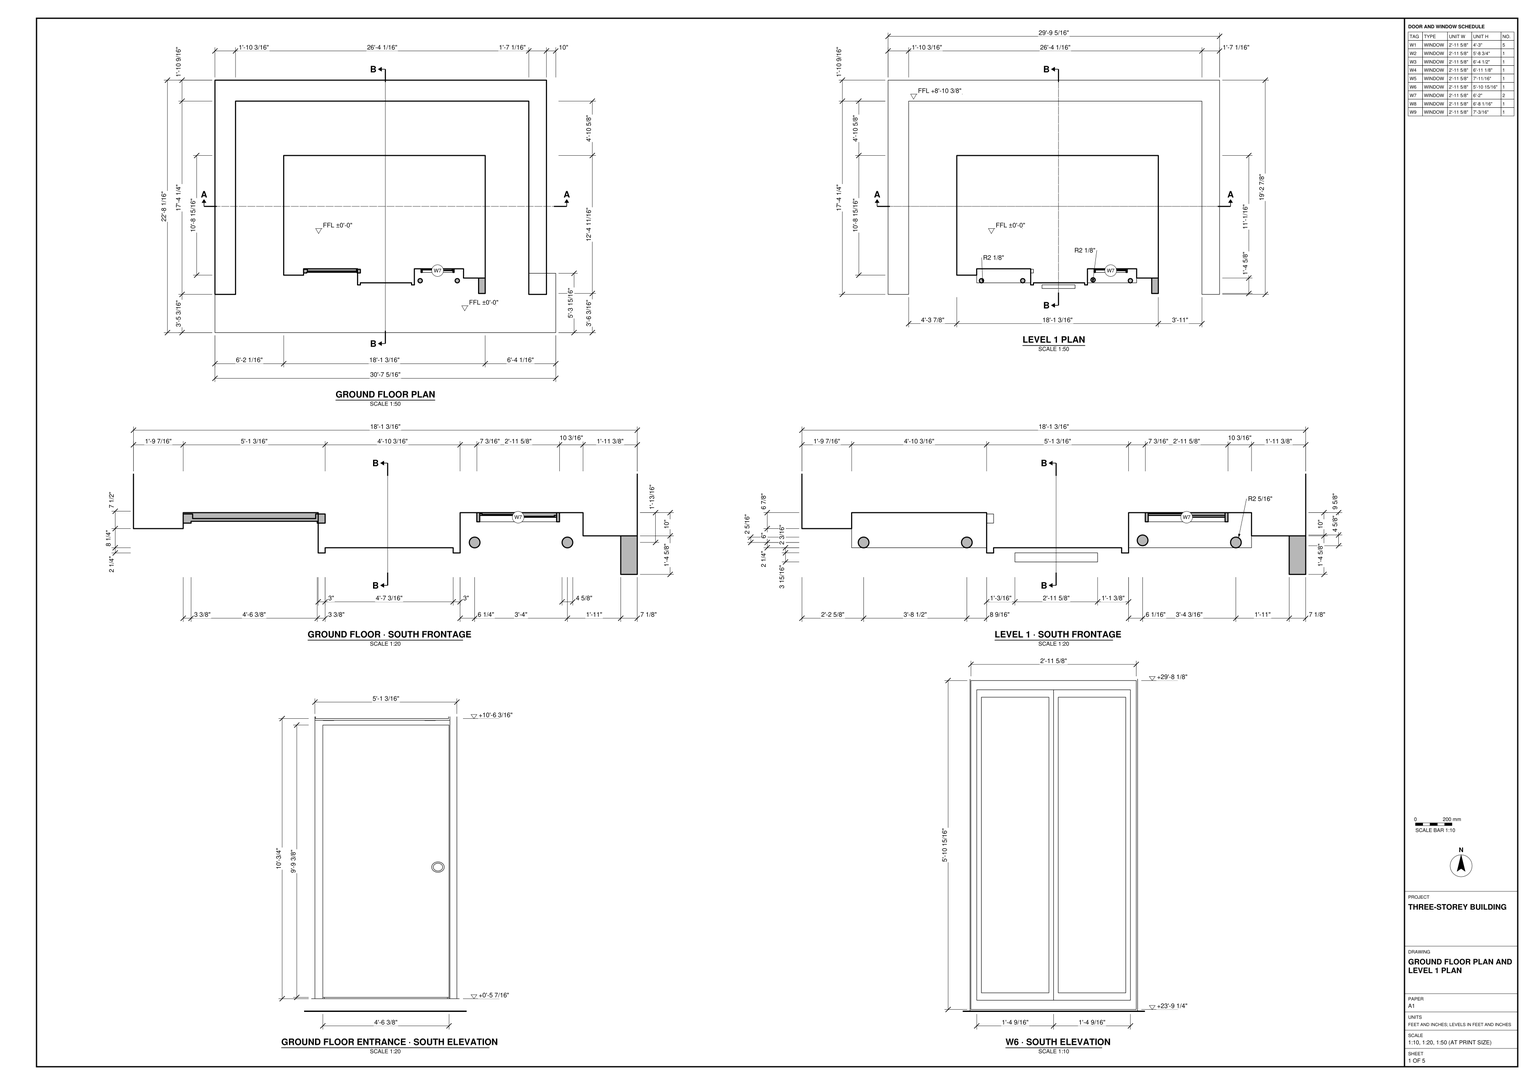
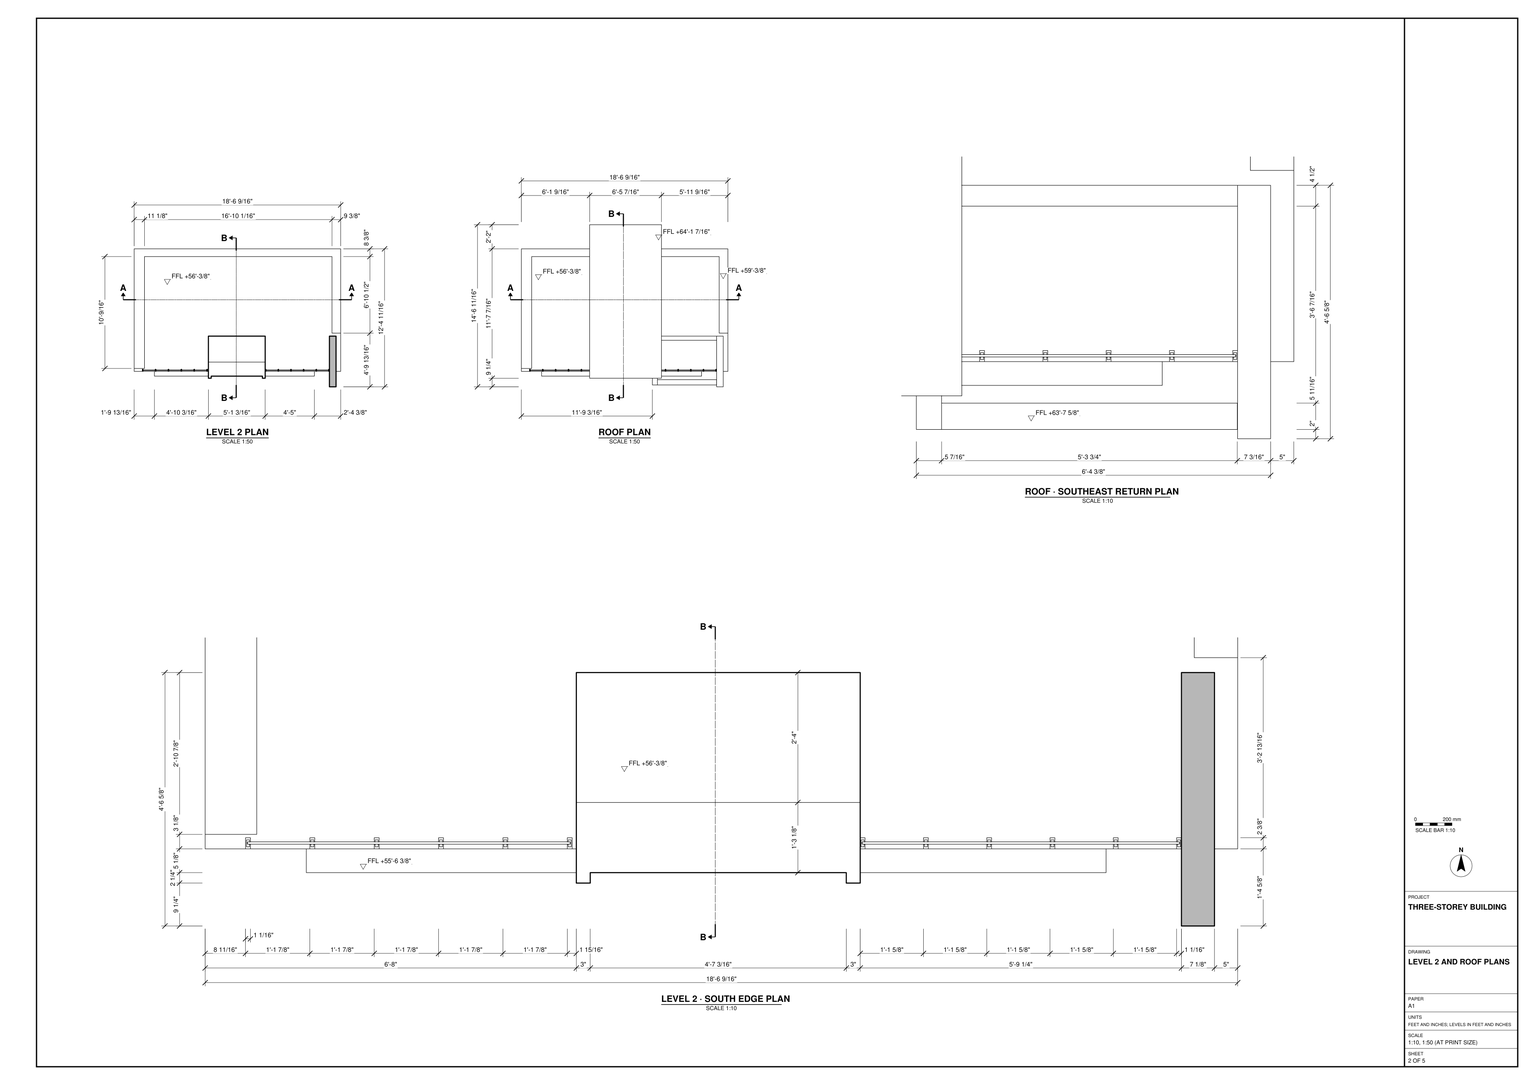
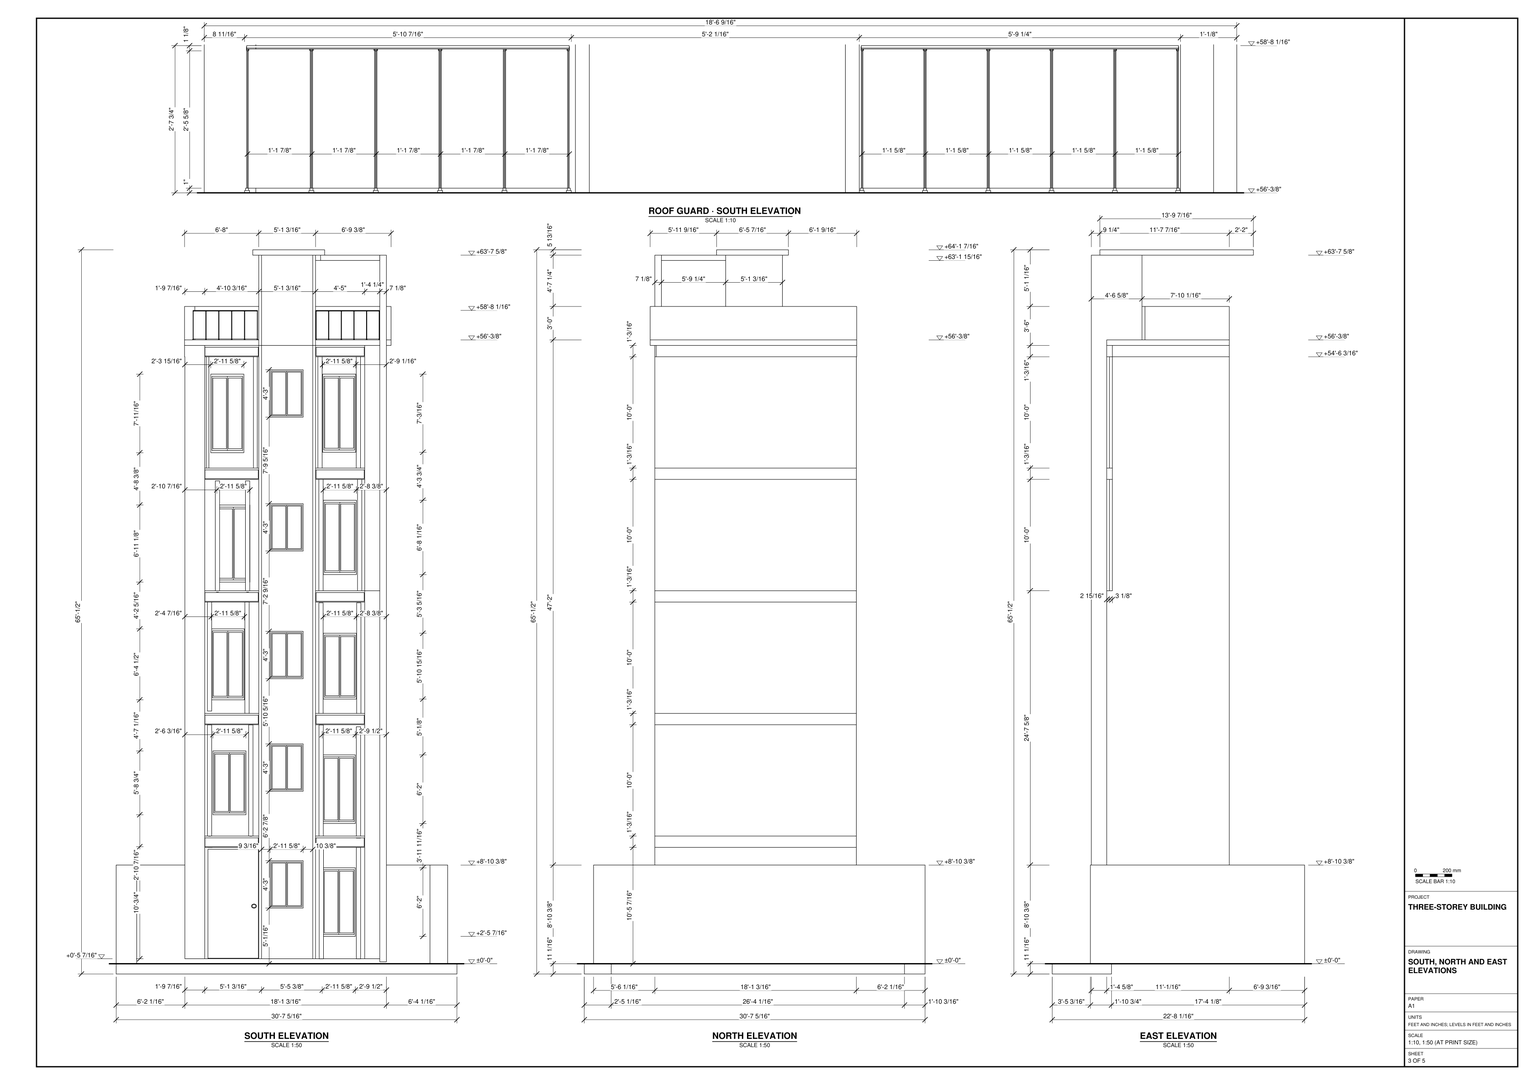
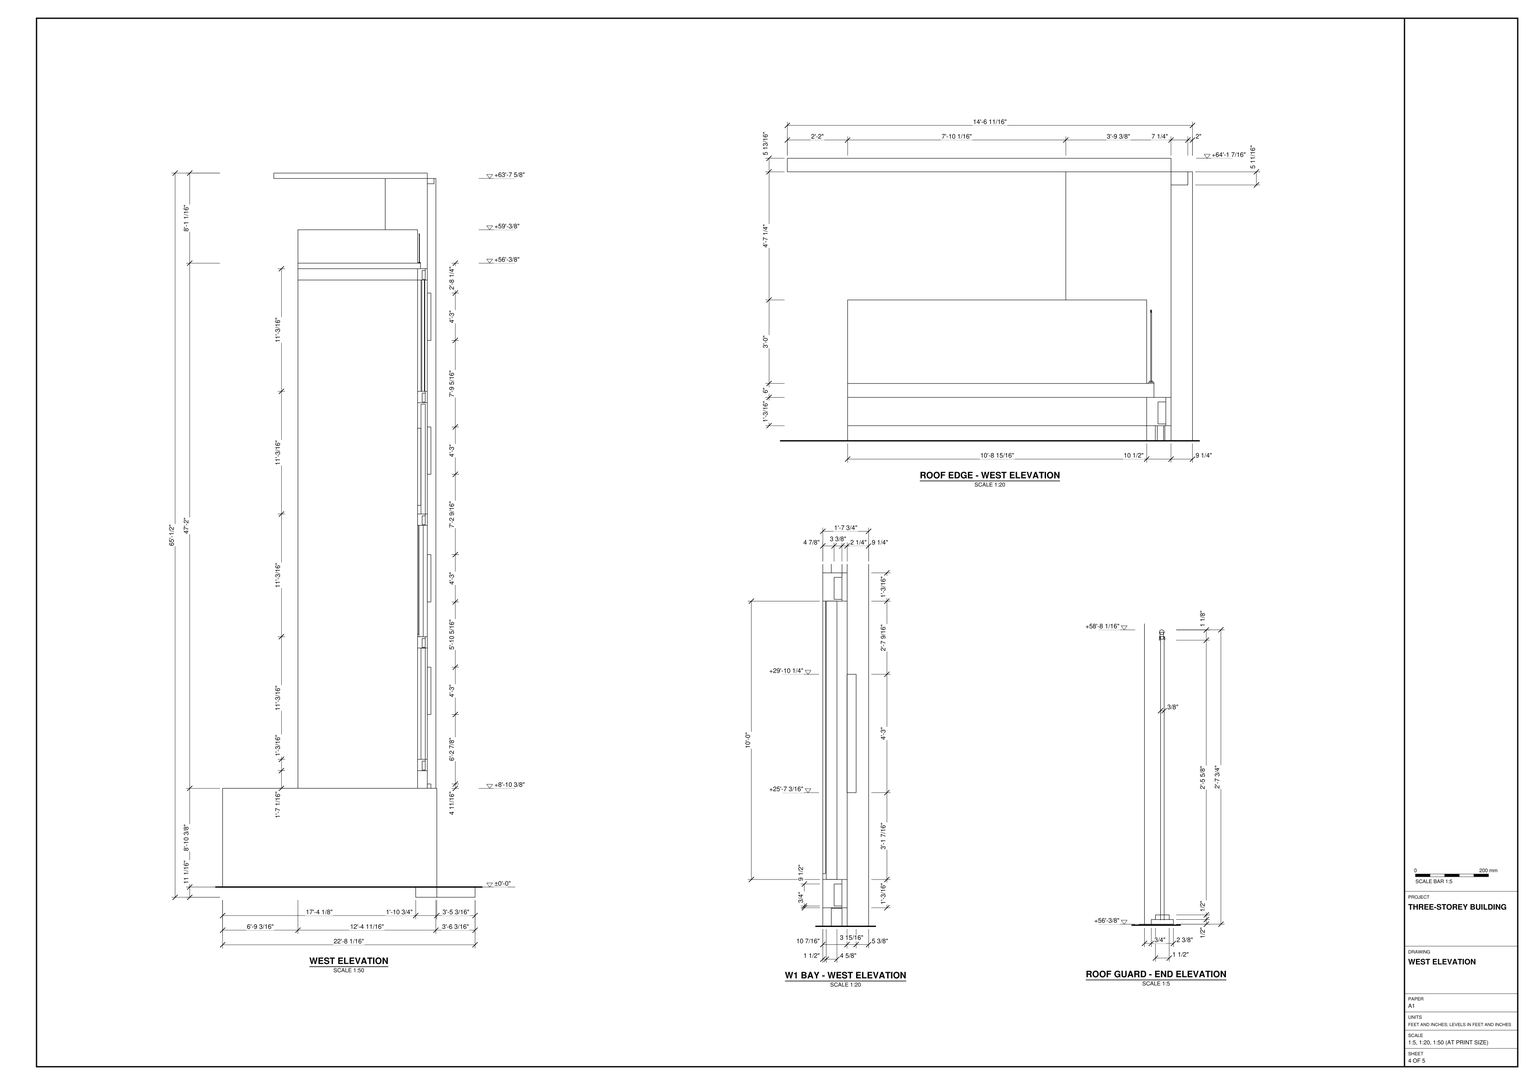
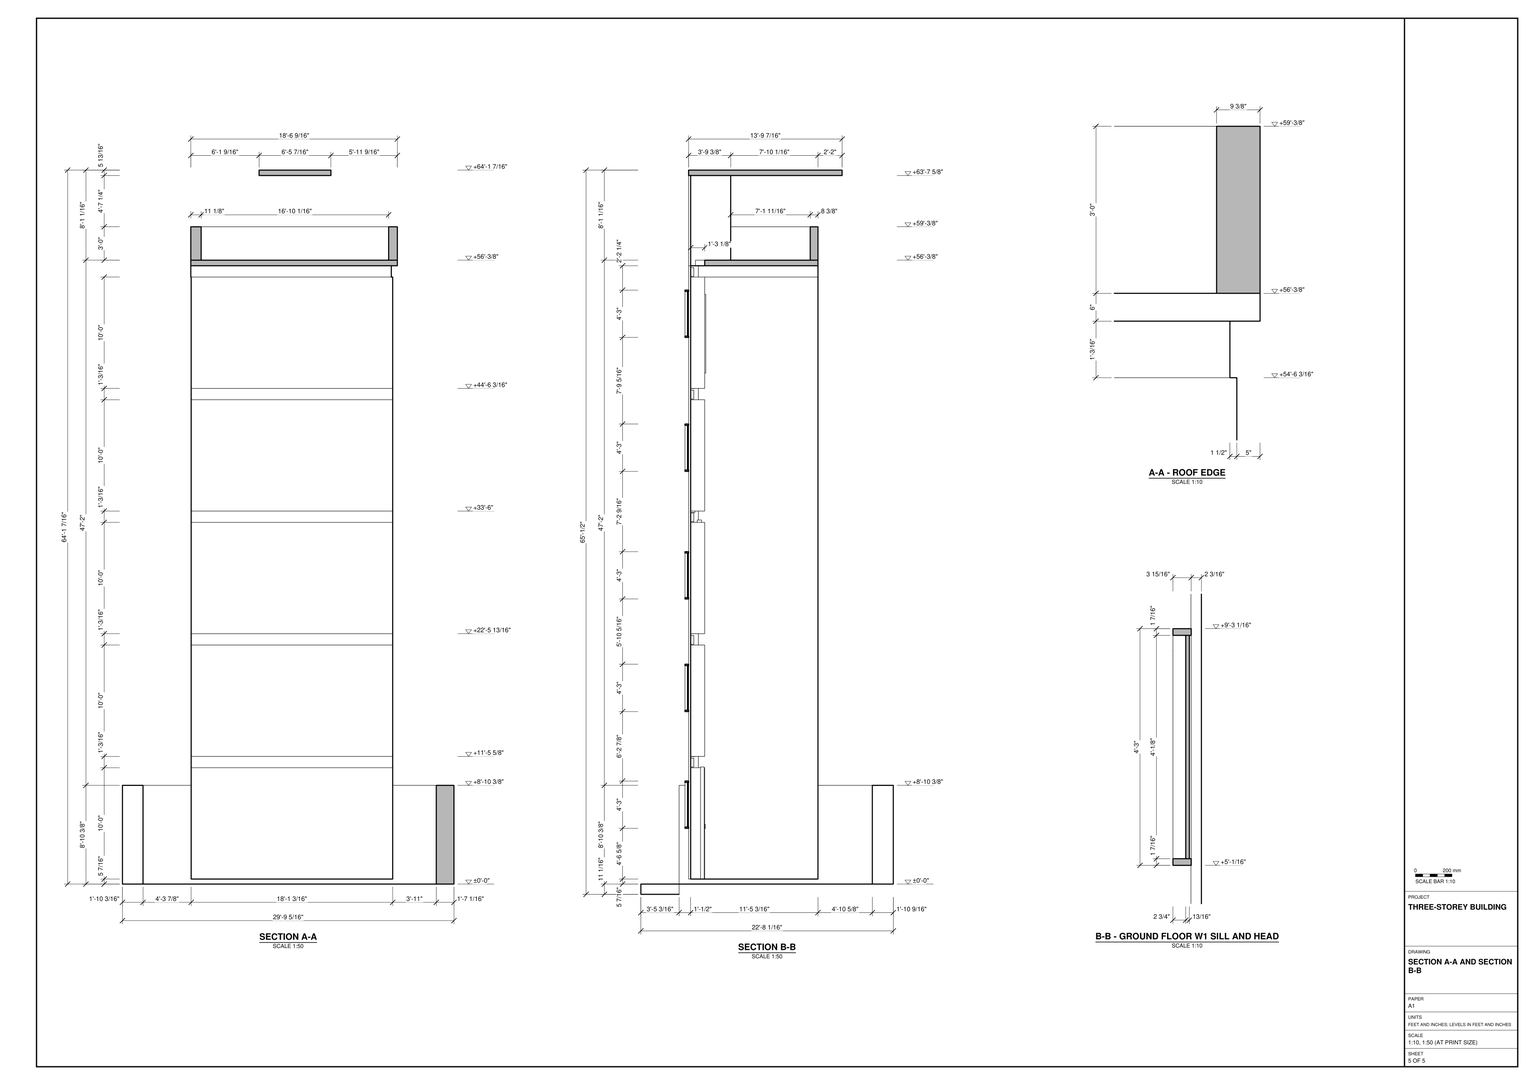
Build the building shown in task_files/diagram_01.pdf in SketchUp. Work in feet and inches. Set the overall width to 30'-7 5/16", the depth to 22'-8 1/16" and the height to 65'-1/2". Use ±0'-0" for the ground floor, +8'-10 3/8" for Level 1 and +56'-3/8" for Level 2.

Start with the ground slab and the U-shaped perimeter wall, leaving the south side open. Position the narrower building block within this surround using the offsets in plan. Follow the drawn wall thicknesses and slab edges. Use the enlarged frontage plans to set the depth of the projecting central bay and the recesses on either side. Place the entrance in the left bay as seen in the south elevation. Match the window rows, sill and head positions, frames and glazing divisions to that elevation. Use the roof plan and southeast return detail to shape the roof overhangs, and fit the glass guards on either side of the raised central bay.

Keep walls, slabs and roof elements in separate groups or components. Keep each furniture or joinery piece shown separate, and use components for repeated parts. Decor and loose items may be any suitable library components. Save one SketchUp model as output_files/three_storey_building_with_a_stepped_south_frontage.skp.

# SketchUp Ruby script. Lengths in inches.
U = 1.inch
M = Sketchup.active_model
def pt(a) = Geom::Point3d.new(a.map { |v| v * U })
def face(e, loops, mat)
  f = e.add_face(loops[0].map { |a| pt(a) })
  loops[1..].each { |l| e.add_face(l.map { |a| pt(a) }).erase! }
  f.material = f.back_material = mat if mat
  f
end
# faces: each face lists its corners as indices into pts; further lists are holes
def faces(e, pts, list, mat = nil) = list.each { |f| face(e, (f[0].is_a?(Array) ? f : [f]).map { |l| l.map { |i| pts[i] } }, mat) }
# xy, xz, yz: faces in a plane at the given z, y or x. An outline is a flat list of corners, or four numbers for a rectangle; further outlines are holes
def ring(l) = l.size == 4 ? [[l[0], l[1]], [l[2], l[1]], [l[2], l[3]], [l[0], l[3]]] : l.each_slice(2).to_a
def flat(e, list, mat, &to3) = list.each { |f| face(e, (f[0].is_a?(Array) ? f : [f]).map { |l| ring(l).map { |u, v| to3.(u, v) } }, mat) }
def xy(e, z, list, mat = nil) = flat(e, list, mat) { |x, y| [x, y, z] }
def xz(e, y, list, mat = nil) = flat(e, list, mat) { |x, z| [x, y, z] }
def yz(e, x, list, mat = nil) = flat(e, list, mat) { |y, z| [x, y, z] }
def lines(e, pts, list) = list.each { |a, b| e.add_line(pt(pts[a]), pt(pts[b])) }
# prism: a flat outline (further loops are holes) pulled along v
def prism(e, loops, v, mat = nil)
  f = face(e, loops, mat); d = Geom::Vector3d.new(v.map { |x| x * U })
  f.pushpull(f.normal.samedirection?(d) ? d.length : -d.length)
end
def box(e, o, s, mat = nil) = prism(e, [[o, [o[0] + s[0], o[1], o[2]], [o[0] + s[0], o[1] + s[1], o[2]], [o[0], o[1] + s[1], o[2]]]], [0, 0, s[2]], mat)
def at(x, y, z, deg = 0) = Geom::Transformation.translation(pt([x, y, z])) * Geom::Transformation.rotation(ORIGIN, Z_AXIS, deg.degrees)
def axes(o, x, y, z) = Geom::Transformation.new([*x, 0, *y, 0, *z, 0, *pt(o).to_a, 1])
def part(name) = M.definitions.add(name)
# library, detail: a bought-in or finely detailed component or shape, given as its bounding box
def library(name, o, s) = part(name).tap { |d| box(d.entities, o, s) }
def detail(e, o, s) = box(e.add_group.entities, o, s)
def put(e, d, t, mat = nil) = e.add_instance(d, t).tap { |i| i.material = mat if mat }
def group(e, t, mat = nil) = e.add_group.tap { |g| g.transformation = t; g.material = mat if mat }.entities
root = M.entities
M.materials.add("[0025_Coral]").color = [255, 127, 80]
M.materials.add("[Roofing Slate Tan]").color = [200, 175, 128]
c1 = library("aluminium+glass+window",[224.88,852.375,0],[3.94,55.9,69.88])
c2 = library("Glass+Railing",[-1.78,-1,-1],[158.25,2.39,31.73])
c3 = library("Group\#9",[0,0,0],[7.48,35.43,84.65])
box(root,[147.28,51.43,763.6],[77.43,165.44,5.81])
prism(root,[[[73.7,61.93,672.35],[73.7,190.87,672.35],[296.28,190.87,672.35],[296.28,100.02,672.35],[286.91,100.02,672.35],[286.91,182.52,672.35],[84.82,182.52,672.35],[84.82,61.93,672.35]]],[0,0,36])
xy(root,-11.0625,[[0,0,367.33,0,367.33,63.9375,338.26,63.9375,338.26,41.1875,0,41.1875]])
xy(root,0,[[0,0,367.33,0,367.33,63.9375,357.3125,63.9375,357.3125,41.1875,338.26,41.1875,338.26,249.47,22.1875,249.47,22.1875,41.1875,0,41.1875],[0,41.1875,0,272.0625,357.3125,272.0625,357.3125,63.9375,338.26,63.9375,338.26,249.47,22.1875,249.47,22.1875,41.1875],[338.26,41.1875,357.3125,63.9375]])
xy(root,106.375,[[0,41.1875,22.1875,41.1875,22.1875,249.47,338.26,249.47,338.26,41.1875,357.3125,41.1875,357.3125,272.0625,0,272.0625]])
xz(root,0,[[0,-11.0625,367.33,0]])
xz(root,41.1875,[[0,-11.0625,22.1875,0],[0,0,22.1875,106.375],[338.26,0,357.3125,106.375]])
xz(root,63.9375,[[338.26,-11.0625,367.33,0]])
xz(root,249.47,[[22.1875,0,338.26,106.375]])
xz(root,272.0625,[[0,0,357.3125,106.375]])
yz(root,0,[[0,-11.0625,41.1875,0],[41.1875,0,272.0625,106.375]])
yz(root,22.1875,[[41.1875,0,249.47,106.375]])
yz(root,338.26,[[41.1875,-11.0625,63.9375,0],[41.1875,0,249.47,106.375]])
yz(root,357.3125,[[41.1875,0,272.0625,106.375]])
yz(root,367.33,[[0,-11.0625,63.9375,0]])
p = [[100.76,58.1875,125.32],[100.2,57.96,125.32],[101.35,58.27,125.32],[99.72,57.59,125.32],[99.35,57.11,125.32],[99.12,56.55,125.32],
  [99.04,55.95,125.32],[99.12,55.36,125.32],[99.35,54.8,125.32],[99.72,54.32,125.32],[100.2,53.95,125.32],[100.76,53.72,125.32],
  [101.35,53.64,125.32],[101.95,53.72,125.32],[102.51,53.95,125.32],[102.99,54.32,125.32],[103.36,54.8,125.32],[103.59,55.36,125.32],
  [103.67,55.95,125.32],[103.59,56.55,125.32],[103.36,57.11,125.32],[102.99,57.59,125.32],[102.51,57.96,125.32],[101.95,58.1875,125.32],
  [146.32,53.95,125.32],[146.8,54.32,125.32],[145.17,58.27,125.32],[144.57,58.1875,125.32],[144.01,57.96,125.32],[143.53,57.59,125.32],
  [143.16,57.11,125.32],[142.93,56.55,125.32],[142.85,55.95,125.32],[142.93,55.36,125.32],[143.16,54.8,125.32],[143.53,54.32,125.32],
  [144.01,53.95,125.32],[144.57,53.72,125.32],[145.17,53.64,125.32],[145.76,53.72,125.32],[147.17,54.8,125.32],[147.4,55.36,125.32],
  [147.48,55.95,125.32],[147.4,56.55,125.32],[147.17,57.11,125.32],[146.8,57.59,125.32],[146.32,57.96,125.32],[145.76,58.1875,125.32]]
lines(root,p,[[0,1],[2,0],[1,3],[3,4],[4,5],[5,6],[6,7],[7,8],[8,9],[9,10],[10,11],[11,12],
  [12,13],[13,14],[14,15],[15,16],[16,17],[17,18],[18,19],[19,20],[20,21],[21,22],[22,23],[23,2],
  [24,25],[26,27],[27,28],[28,29],[29,30],[30,31],[31,32],[32,33],[33,34],[34,35],[35,36],[36,37],
  [37,38],[38,39],[39,24],[25,40],[40,41],[41,42],[42,43],[43,44],[44,45],[45,46],[46,47],[47,26]])
detail(root,[218.46,57.11,401.97],[4.63,4.63,120])
detail(root,[218.46,57.11,269.02],[4.63,4.63,120])
detail(root,[98.35,60.77,272.32],[4.63,4.62,120])
detail(root,[258.76,57.11,534.16],[4.62,4.63,120])
detail(root,[259.21,57.11,269.02],[4.63,4.63,120])
detail(root,[218.85,53.64,5.32],[4.63,4.63,120])
detail(root,[218.64,54.55,137.3],[4.62,4.63,120])
detail(root,[258.85,53.64,135.38],[4.63,4.63,120])
detail(root,[217.38,57.11,534.16],[4.63,4.63,120])
detail(root,[139.35,53.64,400.38],[4.63,4.63,120])
detail(root,[106.85,53.64,400.38],[4.63,4.63,120])
detail(root,[98.35,53.64,137.38],[4.63,4.63,120])
detail(root,[142.85,53.64,137.38],[4.63,4.63,120])
detail(root,[138.73,55.83,269.82],[4.62,4.62,120])
detail(root,[260.15,57.11,401.97],[4.63,4.63,120])
detail(root,[258.85,53.64,5.32],[4.63,4.63,120])
put(root,c1,axes([744.99,-177.33,589.1],[0,1,0],[-0.63756,0,0],[0,0,0.73]))
put(root,c1,axes([744.99,-177.33,60.03],[0,1,0],[-0.63756,0,0],[0,0,0.73]))
put(root,c1,axes([744.99,-177.33,185.91],[0,1,0],[-0.63756,0,0],[0,0,0.73]))
put(root,c1,axes([744.99,-177.33,444.78],[0,1,0],[-0.63756,0,0],[0,0,0.73]))
put(root,c1,axes([744.99,-177.33,307.22],[0,1,0],[-0.63756,0,0],[0,0,0.73]))
put(root,c2,axes([215.69,59.81,673.35],[0.43758,0,0],[0,1,0],[0,0,1]))
put(root,c2,axes([83.19,59.81,673.35],[0.445,0,0],[0,1,0],[0,0,1]))
put(root,c1,axes([801.66,-158.83,551.25],[0,1,0],[-0.63756,0,0],[0,0,1.2045]))
put(root,c1,axes([681.1,-158.83,550.74],[0,1,0],[-0.63756,0,0],[0,0,1.2118]))
put(root,c1,axes([687.625,-166.48,411.24],[0,1,0],[-0.63756,0,0],[0,0,1.1899]))
put(root,c1,axes([802.36,-160.01,419.42],[0,1,0],[-0.63756,0,0],[0,0,1.1461]))
put(root,c1,axes([802.36,-160.01,285.22],[0,1,0],[-0.63756,0,0],[0,0,1.0147]))
put(root,c1,axes([681.61,-160.01,284.41],[0,1,0],[-0.63756,0,0],[0,0,1.095]))
put(root,c1,axes([683.36,-160.01,160.59],[0,1,0],[-0.63756,0,0],[0,0,0.98419]))
put(root,c1,axes([801.1875,-160.01,151.14],[0,1,0],[-0.63756,0,0],[0,0,1.0585]))
put(root,c1,axes([801.1875,-160.01,29.45],[0,1,0],[-0.63756,0,0],[0,0,1.0585]))
g1 = group(root,at(87.07,68.81,5.41))
g2 = group(g1,at(0,-11.1875,0))
g3 = group(g2,at(-13.375,-15.4375,-3.3125))
xy(g3,0,[[210.45,0,217.58,16.625]])
xy(g3,3.3125,[[80.01,9.25,80.01,26.625,21.81,26.625,21.81,19.75,0.375,19.75,0.375,148.69,217.58,148.69,217.58,16.625,194.21,16.625,194.21,26.625,141.21,26.625,141.21,9.25,138.21,9.25,138.21,11.5,83.01,11.5,83.01,9.25]])
xy(g3,123.3125,[[21.81,11.5,80.01,26.625],[141.21,11.5,194.21,26.625]])
xy(g3,124.07,[[22.01,11.5,79.44,14.875]])
xy(g3,124.15,[[141.79,11.5,193.62,15.375]])
xy(g3,133.54,[[141.79,11.5,193.62,15.375]])
xy(g3,133.55,[[22.01,11.5,79.44,14.875]])
xy(g3,135.5,[[21.81,11.5,80.01,26.625],[141.21,11.5,194.21,26.625]])
xy(g3,255.5,[[21.81,11.5,80.01,26.625],[141.21,11.5,194.21,26.625]])
xy(g3,256.26,[[22.01,11.5,79.44,14.875]])
xy(g3,256.34,[[141.79,11.5,193.62,15.375]])
xy(g3,265.73,[[141.79,11.5,193.62,15.375]])
xy(g3,265.74,[[22.01,11.5,79.44,14.875]])
xy(g3,267.6875,[[21.81,11.5,80.01,26.625],[141.21,11.5,194.21,26.625]])
xy(g3,387.6875,[[21.81,11.5,80.01,26.625],[141.21,11.5,194.21,26.625]])
xy(g3,388.45,[[22.01,11.5,79.44,14.875]])
xy(g3,388.52,[[141.79,11.5,193.62,15.375]])
xy(g3,397.91,[[141.79,11.5,193.62,15.375]])
xy(g3,397.93,[[22.01,11.5,79.44,14.875]])
xy(g3,399.875,[[21.81,11.5,80.01,26.625],[141.21,11.5,194.21,26.625],[194.21,16.625,217.58,22.6875]])
xy(g3,519.875,[[21.81,11.5,80.01,26.625],[141.21,11.5,194.21,26.625]])
xy(g3,520.63,[[22.01,11.5,79.44,14.875]])
xy(g3,520.71,[[141.79,11.5,193.62,15.375]])
xy(g3,530.1,[[141.79,11.5,193.62,15.375]])
xy(g3,530.12,[[22.01,11.5,79.44,14.875]])
xy(g3,531.9375,[[76.33,11.91,75.8,11.98,75.3,12.1875,74.875,12.52,74.55,12.94,74.34,13.44,74.27,13.97,74.34,14.51,74.55,15.01,74.875,15.43,75.3,15.76,75.8,15.97,76.33,16.04,76.87,15.97,77.36,15.76,77.79,15.43,78.12,15.01,78.32,14.51,78.39,13.97,78.32,13.44,78.12,12.94,77.79,12.52,77.36,12.1875,76.87,11.98]])
xy(g3,532.0625,[[[21.81,11.5,80.01,26.625],[24.87,12.4375,24.51,12.48,24.18,12.62,23.9,12.84,23.68,13.125,23.54,13.46,23.5,13.8125,23.54,14.17,23.68,14.5,23.9,14.78,24.18,15,24.51,15.14,24.87,15.1875,25.23,15.14,25.56,15,25.84,14.78,26.0625,14.5,26.2,14.17,26.25,13.8125,26.2,13.46,26.0625,13.125,25.84,12.84,25.56,12.62,25.23,12.48]],[141.21,11.5,194.21,26.625]])
xy(g3,652.0625,[[[21.81,11.5,80.01,26.625],[76.33,11.91,76.87,11.98,77.36,12.1875,77.79,12.52,78.12,12.94,78.32,13.44,78.39,13.97,78.32,14.51,78.12,15.01,77.79,15.43,77.36,15.76,76.87,15.97,76.33,16.04,75.8,15.97,75.3,15.76,74.875,15.43,74.55,15.01,74.34,14.51,74.27,13.97,74.34,13.44,74.55,12.94,74.875,12.52,75.3,12.1875,75.8,11.98],[24.87,12.4375,25.23,12.48,25.56,12.62,25.84,12.84,26.0625,13.125,26.2,13.46,26.25,13.8125,26.2,14.17,26.0625,14.5,25.84,14.78,25.56,15,25.23,15.14,24.87,15.1875,24.51,15.14,24.18,15,23.9,14.78,23.68,14.5,23.54,14.17,23.5,13.8125,23.54,13.46,23.68,13.125,23.9,12.84,24.18,12.62,24.51,12.48]],[141.21,11.5,194.21,26.625],[0,19.75,0.375,148.69],[216.08,22.6875,217.58,148.69]])
xy(g3,652.82,[[22.01,11.5,79.44,14.875]])
xy(g3,652.9,[[141.79,11.5,193.62,15.375]])
xy(g3,662.29,[[141.79,11.5,193.62,15.375]])
xy(g3,662.3,[[22.01,11.5,79.44,14.875]])
xy(g3,664.25,[[80.01,9.25,83.01,9.25,83.01,11.5,138.21,11.5,138.21,9.25,141.21,9.25,141.21,26.625,80.01,26.625],[21.81,11.5,80.01,16.625],[141.21,11.5,194.21,16.625],[0,16.625,21.81,19.75],[21.81,16.625,21.81,19.75,0,19.75,0,148.69,216.08,148.69,216.08,22.6875,194.21,22.6875,194.21,16.625,141.21,16.625,141.21,26.625,80.01,26.625,80.01,16.625],
  [194.21,16.625,222.58,22.6875],[216.08,22.6875,222.58,148.69]])
xy(g3,670.25,[[0,16.625,80.01,16.625,80.01,54.625,141.21,54.625,141.21,16.625,210.45,16.625,210.45,54.625,217.58,54.625,217.58,16.625,222.58,16.625,222.58,148.69,0,148.69],[210.45,16.625,217.58,54.625],[80.01,26.625,141.21,54.625]])
xy(g3,755.83,[[141.21,2,141.21,54.625,210.46,54.625,210.46,50.14,146.65,50.14,146.65,2],[146.65,2,210.4,7.67]])
xy(g3,761.5,[[210.45,0,217.58,0,217.58,54.625,210.46,54.625,210.46,50.14,210.45,50.14],[141.21,2,146.65,2,146.65,50.14,210.45,50.14,210.45,54.625,141.21,54.625],[146.65,2,210.4,7.67],[80.01,9.25,83.01,9.25,83.01,11.5,138.21,11.5,138.21,9.25,141.21,9.25,141.21,54.625,80.01,54.625],[210.45,50.14,210.46,54.625]])
xz(g3,0,[[210.45,0,217.58,761.5]])
xz(g3,2,[[141.21,755.83,146.65,761.5],[146.65,755.83,210.4,761.5]])
xz(g3,7.67,[[146.65,755.83,210.4,761.5]])
xz(g3,9.25,[[80.01,3.3125,83.01,664.25],[138.21,3.3125,141.21,664.25],[80.01,664.25,83.01,761.5],[138.21,664.25,141.21,761.5]],"[0025_Coral]")
xz(g3,11.5,[[[21.81,123.3125,80.01,135.5],[22.01,124.07,79.44,133.55]],[[141.21,123.3125,194.21,135.5],[141.79,124.15,193.62,133.54]],[[21.81,255.5,80.01,267.6875],[22.01,256.26,79.44,265.74]],[[141.21,255.5,194.21,267.6875],[141.79,256.34,193.62,265.73]],[[21.81,387.6875,80.01,399.875],[22.01,388.45,79.44,397.93]],
  [[141.21,387.6875,194.21,399.875],[141.79,388.52,193.62,397.91]],[[21.81,519.875,80.01,532.0625],[22.01,520.63,79.44,530.12]],[[141.21,519.875,194.21,532.0625],[141.79,520.71,193.62,530.1]],[[21.81,652.0625,80.01,664.25],[22.01,652.82,79.44,662.3]],[[141.21,652.0625,194.21,664.25],[141.79,652.9,193.62,662.29]]])
xz(g3,11.5,[[83.01,3.3125,138.21,664.25],[83.01,664.25,138.21,761.5]],"[Roofing Slate Tan]")
xz(g3,14.875,[[22.01,124.07,79.44,133.55],[22.01,256.26,79.44,265.74],[22.01,388.45,79.44,397.93],[22.01,520.63,79.44,530.12],[22.01,652.82,79.44,662.3]])
xz(g3,15.375,[[141.79,124.15,193.62,133.54],[141.79,256.34,193.62,265.73],[141.79,388.52,193.62,397.91],[141.79,520.71,193.62,530.1],[141.79,652.9,193.62,662.29]])
xz(g3,16.625,[[210.45,0,217.58,3.3125],[194.21,3.3125,210.45,399.875],[210.45,3.3125,217.58,399.875],[210.45,399.875,217.58,664.25],[0,664.25,80.01,670.25],
  [141.21,664.25,210.45,670.25],[210.45,664.25,217.58,670.25],[217.58,664.25,222.58,670.25]])
xz(g3,19.75,[[0.375,3.3125,21.81,3.3125,21.81,664.25,0,664.25,0,652.0625,0.375,652.0625]])
xz(g3,22.6875,[[194.21,399.875,217.58,399.875,217.58,652.0625,216.08,652.0625,216.08,664.25,194.21,664.25]])
xz(g3,26.625,[[21.81,3.3125,80.01,123.3125],[141.21,3.3125,194.21,123.3125],[21.81,135.5,80.01,255.5],[141.21,135.5,194.21,255.5],[21.81,267.6875,80.01,387.6875],
  [141.21,267.6875,194.21,387.6875],[21.81,399.875,80.01,519.875],[141.21,399.875,194.21,519.875],[21.81,532.0625,80.01,652.0625],[141.21,532.0625,194.21,652.0625],
  [80.01,664.25,141.21,670.25]])
xz(g3,50.14,[[146.65,755.83,210.46,761.5]])
xz(g3,54.625,[[80.01,670.25,141.21,761.5],[210.45,670.25,210.45,755.83,210.46,755.83,210.46,761.5,217.58,761.5,217.58,670.25],[141.21,755.83,210.45,761.5],[210.45,755.83,210.46,761.5]])
xz(g3,148.69,[[0.375,3.3125,217.58,123.3125],[0.375,123.3125,217.58,135.5],[0.375,135.5,217.58,255.5],[0.375,255.5,217.58,267.6875],[0.375,267.6875,217.58,387.6875],
  [0.375,387.6875,217.58,399.875],[0.375,399.875,217.58,519.875],[0.375,519.875,217.58,532.0625],[0.375,532.0625,217.58,652.0625],[0,652.0625,216.08,664.25],
  [0,664.25,222.58,670.25]])
yz(g3,0,[[19.75,652.0625,148.69,664.25],[16.625,664.25,148.69,670.25]])
yz(g3,0.375,[[19.75,3.3125,148.69,652.0625]])
yz(g3,21.81,[[19.75,3.3125,26.625,123.3125],[11.5,123.3125,19.75,135.5],[19.75,135.5,26.625,255.5],[11.5,255.5,19.75,267.6875],[19.75,267.6875,26.625,387.6875],
  [11.5,387.6875,19.75,399.875],[19.75,399.875,26.625,519.875],[11.5,519.875,19.75,532.0625],[19.75,532.0625,26.625,652.0625],[11.5,652.0625,19.75,664.25]])
yz(g3,22.01,[[11.5,124.07,14.875,133.55],[11.5,256.26,14.875,265.74],[11.5,388.45,14.875,397.93],[11.5,520.63,14.875,530.12],[11.5,652.82,14.875,662.3]])
yz(g3,79.44,[[11.5,124.07,14.875,133.55],[11.5,256.26,14.875,265.74],[11.5,388.45,14.875,397.93],[11.5,520.63,14.875,530.12],[11.5,652.82,14.875,662.3]])
yz(g3,80.01,[[9.25,3.3125,26.625,123.3125],[9.25,123.3125,11.5,135.5],[9.25,135.5,26.625,255.5],[9.25,255.5,11.5,267.6875],[9.25,267.6875,26.625,387.6875],
  [9.25,387.6875,11.5,399.875],[9.25,399.875,26.625,519.875],[9.25,519.875,11.5,532.0625],[9.25,532.0625,26.625,652.0625],[9.25,652.0625,11.5,664.25],
  [9.25,664.25,9.25,761.5,54.625,761.5,54.625,670.25,16.625,670.25,16.625,664.25],[16.625,664.25,26.625,670.25]])
yz(g3,83.01,[[9.25,3.3125,11.5,664.25],[9.25,664.25,11.5,761.5]])
yz(g3,138.21,[[9.25,3.3125,11.5,664.25],[9.25,664.25,11.5,761.5]])
yz(g3,141.21,[[9.25,3.3125,26.625,123.3125],[9.25,123.3125,11.5,135.5],[9.25,135.5,26.625,255.5],[9.25,255.5,11.5,267.6875],[9.25,267.6875,26.625,387.6875],
  [9.25,387.6875,11.5,399.875],[9.25,399.875,26.625,519.875],[9.25,519.875,11.5,532.0625],[9.25,532.0625,26.625,652.0625],[9.25,652.0625,11.5,664.25],
  [9.25,664.25,16.625,664.25,16.625,670.25,54.625,670.25,54.625,755.83,9.25,755.83],[16.625,664.25,26.625,670.25],[2,755.83,9.25,761.5],[9.25,755.83,54.625,761.5]])
yz(g3,141.79,[[11.5,124.15,15.375,133.54],[11.5,256.34,15.375,265.73],[11.5,388.52,15.375,397.91],[11.5,520.71,15.375,530.1],[11.5,652.9,15.375,662.29]])
yz(g3,146.65,[[2,755.83,7.67,761.5],[7.67,755.83,50.14,761.5]])
yz(g3,193.62,[[11.5,124.15,15.375,133.54],[11.5,256.34,15.375,265.73],[11.5,388.52,15.375,397.91],[11.5,520.71,15.375,530.1],[11.5,652.9,15.375,662.29]])
yz(g3,194.21,[[16.625,3.3125,26.625,123.3125],[11.5,123.3125,16.625,135.5],[16.625,135.5,26.625,255.5],[11.5,255.5,16.625,267.6875],[16.625,267.6875,26.625,387.6875],
  [11.5,387.6875,16.625,399.875],[22.6875,399.875,26.625,519.875],[11.5,519.875,22.6875,532.0625],[22.6875,532.0625,26.625,652.0625],[11.5,652.0625,22.6875,664.25]])
yz(g3,210.4,[[2,755.83,7.67,761.5]])
yz(g3,210.45,[[0,0,0,761.5,54.625,761.5,54.625,670.25,16.625,670.25,16.625,0]])
yz(g3,210.46,[[50.14,755.83,54.625,761.5]])
yz(g3,216.08,[[22.6875,652.0625,148.69,664.25]])
yz(g3,217.58,[[0,0,16.625,0,16.625,670.25,54.625,670.25,54.625,761.5,0,761.5],[16.625,3.3125,148.69,3.3125,148.69,652.0625,22.6875,652.0625,22.6875,399.875,16.625,399.875]])
yz(g3,222.58,[[16.625,664.25,148.69,670.25]])
p = [[76.33,11.91,652.0625],[75.8,11.98,652.0625],[75.8,11.98,531.9375],[76.33,11.91,531.9375],[76.87,11.98,652.0625],[76.87,11.98,531.9375],
  [75.3,12.1875,652.0625],[75.3,12.1875,531.9375],[77.36,12.1875,652.0625],[77.36,12.1875,531.9375],[74.875,12.52,652.0625],[74.875,12.52,531.9375],
  [77.79,12.52,652.0625],[77.79,12.52,531.9375],[74.55,12.94,652.0625],[74.55,12.94,531.9375],[78.12,12.94,652.0625],[78.12,12.94,531.9375],
  [74.34,13.44,652.0625],[74.34,13.44,531.9375],[78.32,13.44,652.0625],[78.32,13.44,531.9375],[74.27,13.97,652.0625],[74.27,13.97,531.9375],
  [78.39,13.97,652.0625],[78.39,13.97,531.9375],[74.34,14.51,652.0625],[74.34,14.51,531.9375],[78.32,14.51,652.0625],[78.32,14.51,531.9375],
  [74.55,15.01,652.0625],[74.55,15.01,531.9375],[78.12,15.01,652.0625],[78.12,15.01,531.9375],[74.875,15.43,652.0625],[74.875,15.43,531.9375],
  [77.79,15.43,652.0625],[77.79,15.43,531.9375],[75.3,15.76,652.0625],[75.3,15.76,531.9375],[77.36,15.76,652.0625],[77.36,15.76,531.9375],
  [75.8,15.97,652.0625],[75.8,15.97,531.9375],[76.87,15.97,652.0625],[76.87,15.97,531.9375],[76.33,16.04,652.0625],[76.33,16.04,531.9375],
  [24.87,12.4375,652.0625],[24.51,12.48,652.0625],[24.51,12.48,532.0625],[24.87,12.4375,532.0625],[25.23,12.48,652.0625],[25.23,12.48,532.0625],
  [24.18,12.62,652.0625],[24.18,12.62,532.0625],[25.56,12.62,652.0625],[25.56,12.62,532.0625],[23.9,12.84,652.0625],[23.9,12.84,532.0625],
  [25.84,12.84,652.0625],[25.84,12.84,532.0625],[23.68,13.125,652.0625],[23.68,13.125,532.0625],[26.0625,13.125,652.0625],[26.0625,13.125,532.0625],
  [23.54,13.46,652.0625],[23.54,13.46,532.0625],[26.2,13.46,652.0625],[26.2,13.46,532.0625],[23.5,13.8125,652.0625],[23.5,13.8125,532.0625],
  [26.25,13.8125,652.0625],[26.25,13.8125,532.0625],[23.54,14.17,652.0625],[23.54,14.17,532.0625],[26.2,14.17,652.0625],[26.2,14.17,532.0625],
  [23.68,14.5,652.0625],[23.68,14.5,532.0625],[26.0625,14.5,652.0625],[26.0625,14.5,532.0625],[23.9,14.78,652.0625],[23.9,14.78,532.0625],
  [25.84,14.78,652.0625],[25.84,14.78,532.0625],[24.18,15,652.0625],[24.18,15,532.0625],[25.56,15,652.0625],[25.56,15,532.0625],
  [24.51,15.14,652.0625],[24.51,15.14,532.0625],[25.23,15.14,652.0625],[25.23,15.14,532.0625],[24.87,15.1875,652.0625],[24.87,15.1875,532.0625]]
faces(g3,p,[[0,1,2,3],[4,0,3,5],[1,6,7,2],[8,4,5,9],[6,10,11,7],[12,8,9,13],[10,14,15,11],[16,12,13,17],
  [14,18,19,15],[20,16,17,21],[18,22,23,19],[24,20,21,25],[22,26,27,23],[28,24,25,29],[26,30,31,27],[32,28,29,33],
  [30,34,35,31],[36,32,33,37],[34,38,39,35],[40,36,37,41],[38,42,43,39],[44,40,41,45],[42,46,47,43],[46,44,45,47],
  [48,49,50,51],[52,48,51,53],[49,54,55,50],[56,52,53,57],[54,58,59,55],[60,56,57,61],[58,62,63,59],[64,60,61,65],
  [62,66,67,63],[68,64,65,69],[66,70,71,67],[72,68,69,73],[70,74,75,71],[76,72,73,77],[74,78,79,75],[80,76,77,81],
  [78,82,83,79],[84,80,81,85],[82,86,87,83],[88,84,85,89],[86,90,91,87],[92,88,89,93],[90,94,95,91],[94,92,93,95]])
put(root,c3,axes([156.71,61.93,5.41],[0,1,0],[-1.7273,0,0],[0,0,1.42663]))
